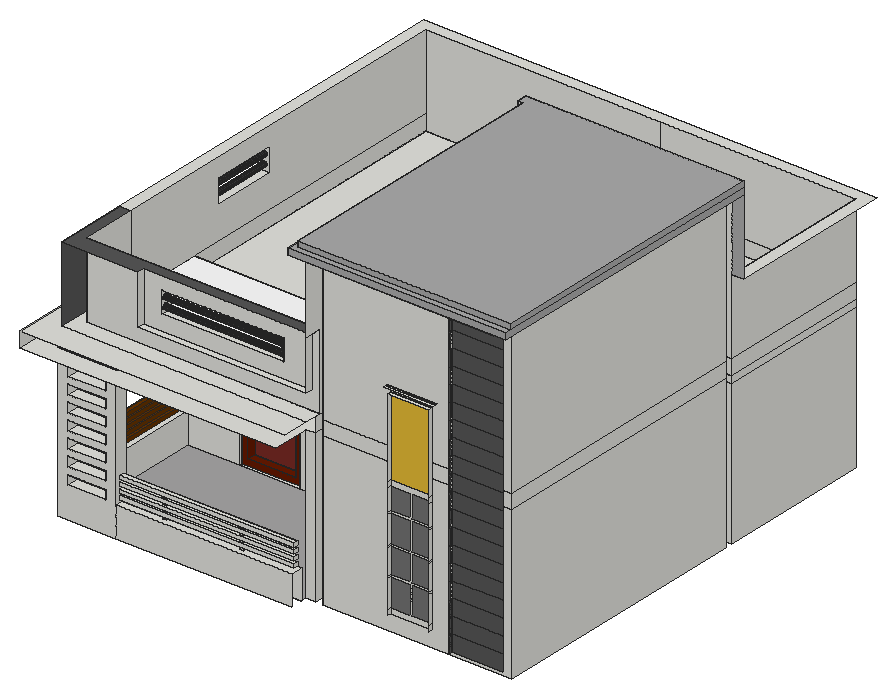
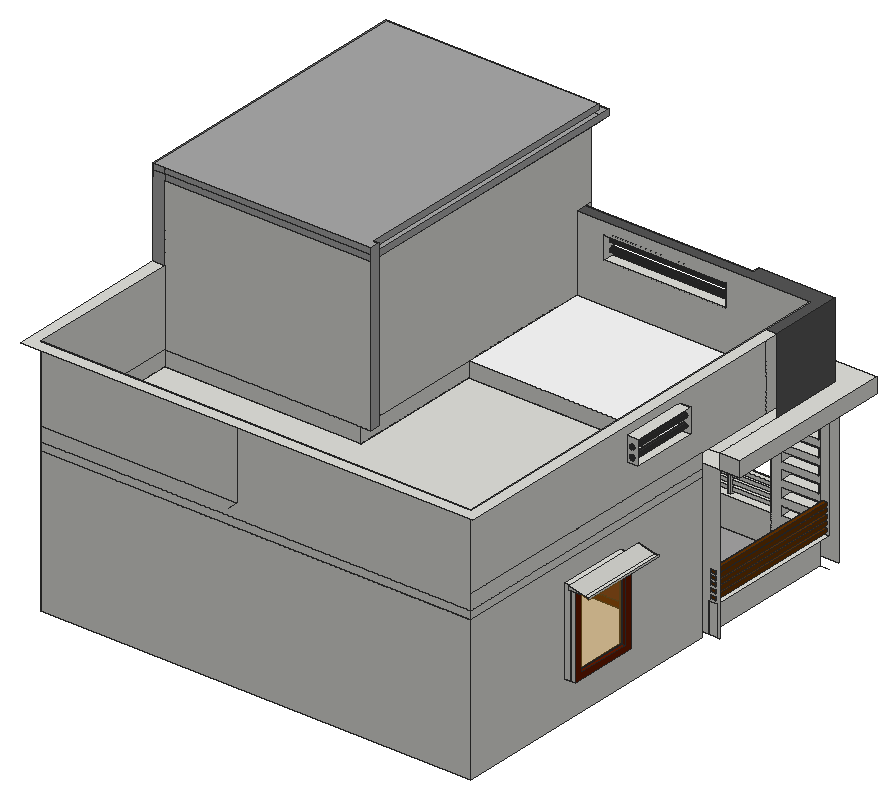
# SketchUp Ruby script. Lengths in inches.
U = 1.inch
M = Sketchup.active_model
def pt(a) = Geom::Point3d.new(a.map { |v| v * U })
def face(e, loops, mat)
  f = e.add_face(loops[0].map { |a| pt(a) })
  loops[1..].each { |l| e.add_face(l.map { |a| pt(a) }).erase! }
  f.material = f.back_material = mat if mat
  f
end
# faces: each face lists its corners as indices into pts; further lists are holes
def faces(e, pts, list, mat = nil) = list.each { |f| face(e, (f[0].is_a?(Array) ? f : [f]).map { |l| l.map { |i| pts[i] } }, mat) }
# xy, xz, yz: faces in a plane at the given z, y or x. An outline is a flat list of corners, or four numbers for a rectangle; further outlines are holes
def ring(l) = l.size == 4 ? [[l[0], l[1]], [l[2], l[1]], [l[2], l[3]], [l[0], l[3]]] : l.each_slice(2).to_a
def flat(e, list, mat, &to3) = list.each { |f| face(e, (f[0].is_a?(Array) ? f : [f]).map { |l| ring(l).map { |u, v| to3.(u, v) } }, mat) }
def xy(e, z, list, mat = nil) = flat(e, list, mat) { |x, y| [x, y, z] }
def xz(e, y, list, mat = nil) = flat(e, list, mat) { |x, z| [x, y, z] }
def yz(e, x, list, mat = nil) = flat(e, list, mat) { |y, z| [x, y, z] }
def lines(e, pts, list) = list.each { |a, b| e.add_line(pt(pts[a]), pt(pts[b])) }
# prism: a flat outline (further loops are holes) pulled along v
def prism(e, loops, v, mat = nil)
  f = face(e, loops, mat); d = Geom::Vector3d.new(v.map { |x| x * U })
  f.pushpull(f.normal.samedirection?(d) ? d.length : -d.length)
end
def box(e, o, s, mat = nil) = prism(e, [[o, [o[0] + s[0], o[1], o[2]], [o[0] + s[0], o[1] + s[1], o[2]], [o[0], o[1] + s[1], o[2]]]], [0, 0, s[2]], mat)
def at(x, y, z, deg = 0) = Geom::Transformation.translation(pt([x, y, z])) * Geom::Transformation.rotation(ORIGIN, Z_AXIS, deg.degrees)
def axes(o, x, y, z) = Geom::Transformation.new([*x, 0, *y, 0, *z, 0, *pt(o).to_a, 1])
def part(name) = M.definitions.add(name)
# library, detail: a bought-in or finely detailed component or shape, given as its bounding box
def library(name, o, s) = part(name).tap { |d| box(d.entities, o, s) }
def detail(e, o, s) = box(e.add_group.entities, o, s)
def put(e, d, t, mat = nil) = e.add_instance(d, t).tap { |i| i.material = mat if mat }
def group(e, t, mat = nil) = e.add_group.tap { |g| g.transformation = t; g.material = mat if mat }.entities
root = M.entities
M.materials.add("[Color B08]").color = [102, 25, 0]
M.materials.add("[Color C08]").color = [102, 51, 0]
M.materials.add("[Color M00]").color = [255, 255, 255]
M.materials.add("[Color M03]").color = [170, 170, 170]
M.materials.add("[Color M05]").color = [114, 114, 114]
M.materials.add("[Color M06]").color = [86, 86, 86]
M.materials.add("[Color M07]").color = [58, 58, 58]
M.materials.add("[Mirror 02]").color = [229, 187, 54]
M.materials.add("[Stone Vein Gray]").color = [166, 165, 165]
M.materials.add("[Translucent Glass Blue]1").color = [223, 149, 22]
M.materials["[Translucent Glass Blue]1"].alpha = 0.5
M.materials.add("[Wood Veneer 01]").color = [120, 43, 37]
c1 = part("Group\#1")
xy(c1.entities,0,[[0,0,48,6.8125]],"[Color B08]")
xy(c1.entities,4.94,[[4.94,0,43.06,6.8125]],"[Color B08]")
xy(c1.entities,79.06,[[4.94,0,43.06,6.8125]],"[Color B08]")
xy(c1.entities,84,[[0,0,48,6.8125]],"[Color B08]")
xz(c1.entities,0,[[[0,0,48,84],[4.94,4.94,43.06,79.06]]],"[Color B08]")
xz(c1.entities,6.8125,[[[0,0,48,84],[4.94,4.94,43.06,79.06]]],"[Color B08]")
xz(c1.entities,6.8125,[[4.94,4.94,43.06,79.06]],"[Wood Veneer 01]")
yz(c1.entities,0,[[0,0,6.8125,84]],"[Color B08]")
yz(c1.entities,4.94,[[0,4.94,6.8125,79.06]],"[Color B08]")
yz(c1.entities,43.06,[[0,4.94,6.8125,79.06]],"[Color B08]")
yz(c1.entities,48,[[0,0,6.8125,84]],"[Color B08]")
c2 = part("Group\#3")
xy(c2.entities,0,[[0,0,48,2.4375]],"[Color B08]")
xy(c2.entities,2.99,[[2.99,0,8.81,2.4375],[8.81,0,14.63,2.4375],[16.47,0,22.65,2.4375],[22.65,0,28.82,2.4375],[30.66,0,45.01,2.4375]],"[Color B08]")
xy(c2.entities,57.01,[[2.99,0,8.81,2.4375],[8.81,0,14.63,2.4375],[16.47,0,22.65,2.4375],[22.65,0,28.82,2.4375],[30.66,0,45.01,2.4375]],"[Color B08]")
xy(c2.entities,60,[[0,0,48,2.4375]],"[Color B08]")
xz(c2.entities,0,[[[0,0,48,60],[30.66,2.99,45.01,57.01],[16.47,2.99,28.82,57.01],[2.99,2.99,14.63,57.01]]],"[Color B08]")
xz(c2.entities,2.4375,[[[0,0,48,60],[30.66,2.99,45.01,57.01],[16.47,2.99,28.82,57.01],[2.99,2.99,14.63,57.01]]],"[Color B08]")
xz(c2.entities,2.4375,[[2.99,2.99,8.81,57.01],[8.81,2.99,14.63,57.01],[16.47,2.99,22.65,57.01],[22.65,2.99,28.82,57.01],[30.66,2.99,45.01,57.01]],"[Translucent Glass Blue]1")
yz(c2.entities,0,[[0,0,2.4375,60]],"[Color B08]")
yz(c2.entities,2.99,[[0,2.99,2.4375,57.01]],"[Color B08]")
yz(c2.entities,14.63,[[0,2.99,2.4375,57.01]],"[Color B08]")
yz(c2.entities,16.47,[[0,2.99,2.4375,57.01]],"[Color B08]")
yz(c2.entities,28.82,[[0,2.99,2.4375,57.01]],"[Color B08]")
yz(c2.entities,30.66,[[0,2.99,2.4375,57.01]],"[Color B08]")
yz(c2.entities,45.01,[[0,2.99,2.4375,57.01]],"[Color B08]")
yz(c2.entities,48,[[0,0,2.4375,60]],"[Color B08]")
c3 = part("Group\#2")
xy(c3.entities,0,[[0,0,23.0625,1.75]],"[Color B08]")
xy(c3.entities,2.13,[[2.13,0,20.93,1.75]],"[Color B08]")
xy(c3.entities,29.8,[[2.13,0,20.93,1.75]],"[Color B08]")
xy(c3.entities,31.9375,[[0,0,23.0625,1.75]],"[Color B08]")
xz(c3.entities,0,[[[0,0,23.0625,31.9375],[2.13,2.13,20.93,29.8]]],"[Color B08]")
xz(c3.entities,1.75,[[[0,0,23.0625,31.9375],[2.13,2.13,20.93,29.8]]],"[Color B08]")
xz(c3.entities,1.75,[[2.13,2.13,20.93,29.8]],"[Translucent Glass Blue]1")
yz(c3.entities,0,[[0,0,1.75,31.9375]],"[Color B08]")
yz(c3.entities,2.13,[[0,2.13,1.75,29.8]],"[Color B08]")
yz(c3.entities,20.93,[[0,2.13,1.75,29.8]],"[Color B08]")
yz(c3.entities,23.0625,[[0,0,1.75,31.9375]],"[Color B08]")
box(root,[62.5625,70.38,249.27],[140.5,3.75,3])
xy(root,213,[[65.72,188.125,113.72,194.125]])
xy(root,213,[[24.85,77.25,203.0625,77.25,203.0625,82.125,210.75,82.125,210.75,188.125,24.85,188.125]],"[Stone Vein Gray]")
xy(root,237,[[[64.19,67.5,203.8125,77.25],[97.86,71.77,100.86,74.2],[158.98,71.77,161.98,74.14]],[97.86,71.77,100.86,74.2],[158.98,71.77,161.98,74.14],[17.6875,77.25,24.85,188.125]])
xy(root,237.55,[[25.89,67.5,55.51,77.25]])
xy(root,239.03,[[19.03,76.6875,22.65,188.125]],"[Color C08]")
xy(root,239.52,[[64.19,70.38,203.0625,74.13]])
xy(root,241.59,[[134.6,188.125,182.6,194.125]])
xy(root,242.03,[[19.03,76.6875,22.65,188.125]],"[Color C08]")
xy(root,242.52,[[64.19,70.38,203.0625,74.13]])
xy(root,243.91,[[19.03,76.375,22.65,188.125]],"[Color C08]")
xy(root,244.22,[[16.0625,276.01,25.0625,331.39]])
xy(root,244.4,[[64.19,70.38,203.0625,74.13]])
xy(root,245.23,[[25.89,67.5,55.51,77.25]])
xy(root,246.91,[[19.03,76.375,22.65,188.125]],"[Color C08]")
xy(root,247.4,[[64.19,70.38,203.0625,74.13]])
xy(root,248.53,[[19.03,77.0625,22.65,188.125]],"[Color C08]")
xy(root,250.86,[[25.89,67.5,55.51,77.25]])
xy(root,251.53,[[19.03,77.0625,22.65,188.125]],"[Color C08]")
xy(root,253.22,[[19.03,77.0625,22.65,188.125]],"[Color C08]")
xy(root,254.15,[[64.19,70.38,64.19,74.13,97.86,74.13,97.86,71.77,100.86,71.77,100.86,74.13,158.98,74.13,158.98,71.77,161.98,71.77,161.98,74.13,203.0625,74.13,203.0625,70.38],[97.86,71.77,100.86,74.13],[158.98,71.77,161.98,74.13],[97.86,74.13,100.86,74.2],[158.98,74.13,161.98,74.14]])
xy(root,256.22,[[19.03,77.0625,22.65,188.125]],"[Color C08]")
xy(root,257.15,[[64.19,70.38,203.0625,74.13]])
xy(root,257.53,[[19.03,76.6875,22.65,188.125]],"[Color C08]")
xy(root,258.55,[[25.89,67.5,55.51,77.25]])
xy(root,260.53,[[19.03,76.6875,22.65,188.125]],"[Color C08]")
xy(root,263.67,[[25.89,67.5,55.51,77.25]])
xy(root,271.36,[[25.89,67.5,55.51,77.25]])
xy(root,276.48,[[25.89,67.5,55.51,77.25]])
xy(root,284.17,[[25.89,67.5,55.51,77.25]])
xy(root,289.3,[[25.89,67.5,55.51,77.25]])
xy(root,296.98,[[25.89,67.5,55.51,77.25]])
xy(root,297,[[65.72,188.125,113.72,194.125]])
xy(root,301.59,[[134.6,188.125,182.6,194.125]])
xy(root,302.11,[[25.89,67.5,55.51,77.25]])
xy(root,309.8,[[25.89,67.5,55.51,77.25]])
xy(root,312.41,[[16.0625,276.01,25.0625,331.39]])
xy(root,313.31,[[0,268.71,16.0625,338.34]])
xy(root,314.92,[[25.89,67.5,55.51,77.25]])
xy(root,322.61,[[25.89,67.5,55.51,77.25]])
xy(root,327,[[25.0625,194.125,25.0625,424.125,367.0625,424.125,367.0625,300.9375,210.75,300.9375,210.75,194.125]])
xy(root,333,[[[0.0625,52.25,0.0625,188.125,210.75,188.125,210.75,82.125,203.0625,82.125,203.0625,52.25],[17.6875,67.5,64.19,77.25]],[17.6875,67.5,25.0625,77.25],[25.0625,67.5,64.19,77.25],[25.0625,194.125,210.75,194.125,210.75,300.9375,367.0625,300.9375,367.0625,424.125,25.0625,424.125]])
xy(root,345,[[0.0625,52.25,210.75,52.25,210.75,73.125,16.0625,73.125,16.0625,188.125,0.0625,188.125],[16.0625,73.125,210.75,73.125,210.75,87.0625,25.0625,87.0625,25.0625,188.125,16.0625,188.125],[203.125,292.82,210.75,300.9375]])
xy(root,345,[[25.0625,87.0625,210.75,194.125]],"[Color M00]")
xy(root,365.8125,[[77.05,73.125,210.75,78.37]])
xy(root,371.23,[[16.0625,216.9,25.0625,269.27]])
xy(root,377.7,[[91.9,78.37,188.65,87.0625]])
xy(root,390.23,[[16.0625,216.9,25.0625,269.27]])
xy(root,391.56,[[279.64,68.125,312.19,71.0625]])
xy(root,395.03,[[276.17,68.125,315.67,70.125],[276.17,70.125,315.67,71.0625]])
xy(root,395.03,[[276.17,71.0625,315.67,72]],"[Color M06]")
xy(root,395.14,[[91.9,78.37,188.65,87.0625]])
xy(root,405,[[16.0625,130.91,25.0625,130.91,25.0625,424.125,367.0625,424.125,367.0625,300.9375,376.0625,300.9375,376.0625,433.125,16.0625,433.125]])
xy(root,405,[[16.0625,73.125,77.05,73.125,77.05,78.37,210.75,78.37,210.75,87.0625,25.0625,87.0625,25.0625,130.91,16.0625,130.91]],"[Color M06]")
xy(root,459,[[216.75,82.125,367.0625,294.9375]])
xy(root,465,[[203.125,64.625,203.125,73.125,264.41,73.125,264.41,70.125,326.55,70.125,326.55,73.125,367.0625,73.125,367.0625,64.625],[264.41,70.125,326.55,71.0625],[264.41,72,326.55,73.125],[216.75,82.125,367.0625,294.9375],[216.75,82.125,367.0625,294.9375]])
xy(root,465,[[203.125,73.125,210.75,292.82]],"[Color M03]")
xy(root,465,[[264.41,71.0625,326.55,72]],"[Color M06]")
xy(root,470,[[203.125,64.625,376.0625,64.625,376.0625,69.375,207.125,69.375,207.125,73.125,203.125,73.125],[203.125,73.125,207.125,292.82]],"[Color M03]")
xy(root,474.75,[[207.125,69.375,376.0625,69.375,376.0625,300.9375,203.125,300.9375,203.125,292.82,207.125,292.82]],"[Color M03]")
xz(root,64.625,[[203.125,465,376.0625,470]],"[Color M03]")
xz(root,67.5,[[[17.6875,213,64.19,333],[25.89,314.92,55.51,322.61],[25.89,302.11,55.51,309.8],[25.89,289.3,55.51,296.98],[25.89,276.48,55.51,284.17],[25.89,263.67,55.51,271.36],[25.89,250.86,55.51,258.55],[25.89,237.55,55.51,245.23]],[64.19,213,203.8125,237]])
xz(root,69.375,[[207.125,470,376.0625,474.75]],"[Color M03]")
xz(root,70.38,[[64.19,239.52,203.0625,242.52],[64.19,244.4,203.0625,247.4],[64.19,254.15,203.0625,257.15]])
xz(root,71.0625,[[279.64,233.67,312.19,233.67,312.19,237.9,296.12,237.9,296.12,260.0625,312.19,260.0625,312.19,261.53,296.12,261.53,296.12,282,312.19,282,312.19,283.47,296.12,283.47,296.12,305.625,312.19,305.625,312.19,307.09,296.12,307.09,296.12,324.48,312.19,324.48,312.19,328.71,279.64,328.71,279.64,324.48,295.68,324.48,295.68,307.09,279.64,307.09,279.64,305.625,295.68,305.625,295.68,283.47,279.64,283.47,279.64,282,295.68,282,295.68,261.53,279.64,261.53,279.64,260.0625,295.68,260.0625,295.68,237.9,279.64,237.9]])
xz(root,71.0625,[[279.64,237.9,295.68,260.0625],[296.12,237.9,312.19,260.0625],[279.64,261.53,295.68,282],[296.12,261.53,312.19,282],[279.64,283.47,295.68,305.625],
  [296.12,283.47,312.19,305.625],[279.64,307.09,295.68,324.48],[296.12,307.09,312.19,324.48]],"[Color M05]")
xz(root,71.0625,[[279.64,328.71,312.19,391.56]],"[Mirror 02]")
xz(root,71.77,[[97.86,237,100.86,254.15],[158.98,237,161.98,254.15]])
xz(root,73.125,[[326.55,221.85,367.0625,234.6],[326.55,234.6,367.0625,247.35],[326.55,247.35,367.0625,260.1],[326.55,260.1,367.0625,272.85],[326.55,272.85,367.0625,285.6],
  [326.55,285.6,367.0625,298.35],[326.55,298.35,367.0625,311.1],[326.55,311.1,367.0625,323.85],[326.55,323.85,367.0625,336.6],[326.55,336.6,367.0625,349.35],
  [326.55,349.35,367.0625,362.1],[326.55,362.1,367.0625,374.85],[326.55,374.85,367.0625,387.6],[326.55,387.6,367.0625,400.35],[326.55,400.35,367.0625,413.1],
  [326.55,413.1,367.0625,425.85],[326.55,425.85,367.0625,438.6],[326.55,438.6,367.0625,451.35],[326.55,451.35,367.0625,465]],"[Color M06]")
xz(root,74.13,[[64.19,239.52,203.0625,242.52],[64.19,244.4,203.0625,247.4],[64.19,254.15,203.0625,257.15]])
xz(root,74.14,[[158.98,237,161.98,254.15]])
xz(root,74.2,[[97.86,237,100.86,254.15]])
xz(root,76.375,[[19.03,243.91,22.65,246.91]],"[Color C08]")
xz(root,76.6875,[[19.03,239.03,22.65,242.03],[19.03,257.53,22.65,260.53]],"[Color C08]")
xz(root,77.0625,[[19.03,248.53,22.65,251.53],[19.03,253.22,22.65,256.22]],"[Color C08]")
xz(root,77.25,[[[24.85,213,64.19,333],[25.89,314.92,55.51,322.61],[25.89,302.11,55.51,309.8],[25.89,289.3,55.51,296.98],[25.89,276.48,55.51,284.17],[25.89,263.67,55.51,271.36],[25.89,250.86,55.51,258.55],[25.89,237.55,55.51,245.23]],[64.19,213,203.8125,237],[17.6875,237,24.85,333]])
xz(root,78.37,[[[77.05,365.8125,210.75,405],[91.9,377.7,188.65,395.14]]])
xz(root,82.125,[[203.0625,213,210.75,333],[216.75,213,367.0625,333],[216.75,333,367.0625,345],[216.75,345,367.0625,459],[216.75,459,367.0625,465]])
xz(root,87.0625,[[[25.0625,345,210.75,405],[91.9,377.7,188.65,395.14]]])
xz(root,188.125,[[[16.0625,213,17.6875,213,17.6875,237,24.85,237,24.85,213,65.72,213,65.72,297,113.72,297,113.72,213,210.75,213,210.75,333,16.0625,333],[134.6,241.59,182.6,301.59],[19.03,257.53,22.65,260.53],[19.03,253.22,22.65,256.22],[19.03,248.53,22.65,251.53],[19.03,243.91,22.65,246.91],[19.03,239.03,22.65,242.03]],[17.6875,213,24.85,237],[0.0625,333,16.0625,345]])
xz(root,188.125,[[19.03,239.03,22.65,242.03],[19.03,243.91,22.65,246.91],[19.03,248.53,22.65,251.53],[19.03,253.22,22.65,256.22],[19.03,257.53,22.65,260.53]],"[Color C08]")
xz(root,194.125,[[[25.0625,213,25.0625,327,210.75,327,210.75,213,113.72,213,113.72,297,65.72,297,65.72,213],[134.6,241.59,182.6,301.59]],[25.0625,327,133.62,333],[133.62,327,144.06,333],[144.06,327,210.75,333],[25.0625,333,210.75,345]])
xz(root,216.27,[[20.63,373.94,21.15,374.01,21.63,374.21,22.05,374.53,22.36,374.94,22.5625,375.42,22.63,375.94,22.5625,376.46,22.36,376.94,22.05,377.35,21.63,377.67,21.15,377.87,20.63,377.94,20.11,377.87,19.63,377.67,19.22,377.35,18.9,376.94,18.7,376.46,18.63,375.94,18.7,375.42,18.9,374.94,19.22,374.53,19.63,374.21,20.11,374.01]],"[Color M07]")
xz(root,216.9,[[[16.0625,371.23,25.0625,390.23],[20.63,381.38,21.15,381.45,21.63,381.65,22.05,381.96,22.36,382.38,22.5625,382.86,22.63,383.38,22.5625,383.9,22.36,384.38,22.05,384.79,21.63,385.11,21.15,385.31,20.63,385.38,20.11,385.31,19.63,385.11,19.22,384.79,18.9,384.38,18.7,383.9,18.63,383.38,18.7,382.86,18.9,382.38,19.22,381.96,19.63,381.65,20.11,381.45]]])
xz(root,268.71,[[0,312.33,0,313.31,16.0625,313.31,16.0625,316.56,3.71,313.31]])
xz(root,269.27,[[[16.0625,371.23,25.0625,390.23],[20.63,373.94,20.11,374.01,19.63,374.21,19.22,374.53,18.9,374.94,18.7,375.42,18.63,375.94,18.7,376.46,18.9,376.94,19.22,377.35,19.63,377.67,20.11,377.87,20.63,377.94,21.15,377.87,21.63,377.67,22.05,377.35,22.36,376.94,22.5625,376.46,22.63,375.94,22.5625,375.42,22.36,374.94,22.05,374.53,21.63,374.21,21.15,374.01],[20.63,381.38,20.11,381.45,19.63,381.65,19.22,381.96,18.9,382.38,18.7,382.86,18.63,383.38,18.7,383.9,18.9,384.38,19.22,384.79,19.63,385.11,20.11,385.31,20.63,385.38,21.15,385.31,21.63,385.11,22.05,384.79,22.36,384.38,22.5625,383.9,22.63,383.38,22.5625,382.86,22.36,382.38,22.05,381.96,21.63,381.65,21.15,381.45]]])
xz(root,269.27,[[20.63,373.94,20.11,374.01,19.63,374.21,19.22,374.53,18.9,374.94,18.7,375.42,18.63,375.94,18.7,376.46,18.9,376.94,19.22,377.35,19.63,377.67,20.11,377.87,20.63,377.94,21.15,377.87,21.63,377.67,22.05,377.35,22.36,376.94,22.5625,376.46,22.63,375.94,22.5625,375.42,22.36,374.94,22.05,374.53,21.63,374.21,21.15,374.01],[20.63,381.38,20.11,381.45,19.63,381.65,19.22,381.96,18.9,382.38,18.7,382.86,18.63,383.38,18.7,383.9,18.9,384.38,19.22,384.79,19.63,385.11,20.11,385.31,20.63,385.38,21.15,385.31,21.63,385.11,22.05,384.79,22.36,384.38,22.5625,383.9,22.63,383.38,22.5625,382.86,22.36,382.38,22.05,381.96,21.63,381.65,21.15,381.45]],"[Color M07]")
xz(root,276.01,[[16.0625,244.22,25.0625,312.41]])
xz(root,292.82,[[203.125,470,207.125,474.75]])
xz(root,292.82,[[203.125,345,210.75,465]],"[Color M03]")
xz(root,294.9375,[[216.75,213,367.0625,333],[216.75,333,367.0625,345],[216.75,345,367.0625,459],[216.75,459,266.67,465],[266.67,459,311.1,465],
  [311.1,459,367.0625,465]])
xz(root,300.9375,[[210.75,213,367.0625,327],[210.75,327,367.0625,333],[210.75,333,367.0625,345],[203.125,345,367.0625,465]])
xz(root,300.9375,[[367.0625,405,376.0625,470],[203.125,465,367.0625,470],[203.125,470,367.0625,474.75],[367.0625,470,376.0625,474.75]],"[Color M03]")
xz(root,331.39,[[16.0625,244.22,25.0625,312.41]])
xz(root,338.34,[[0,312.33,3.71,313.31,16.0625,316.56,16.0625,313.31,0,313.31]])
xz(root,424.125,[[25.0625,213,367.0625,327],[25.0625,327,367.0625,333],[25.0625,333,367.0625,333,367.0625,345,210.75,345,210.75,405,25.0625,405],[210.75,345,367.0625,405]])
yz(root,0,[[268.71,312.33,338.34,313.31]])
yz(root,0.0625,[[52.25,333,188.125,345]])
yz(root,16.0625,[[73.125,345,130.91,405]],"[Color M06]")
yz(root,19.03,[[76.6875,239.03,188.125,242.03],[76.375,243.91,188.125,246.91],[77.0625,248.53,188.125,251.53],[77.0625,253.22,188.125,256.22],[76.6875,257.53,188.125,260.53]],"[Color C08]")
yz(root,22.65,[[76.6875,239.03,188.125,242.03],[76.375,243.91,188.125,246.91],[77.0625,248.53,188.125,251.53],[77.0625,253.22,188.125,256.22],[76.6875,257.53,188.125,260.53]],"[Color C08]")
yz(root,24.85,[[77.25,213,188.125,237]])
yz(root,25.0625,[[[194.125,213,424.125,327],[276.01,244.22,331.39,312.41]],[194.125,327,424.125,333],[194.125,333,424.125,345],[87.0625,345,130.91,405],[[130.91,345,424.125,405],[216.9,371.23,269.27,390.23]]])
yz(root,25.89,[[67.5,237.55,77.25,245.23],[67.5,250.86,77.25,258.55],[67.5,263.67,77.25,271.36],[67.5,276.48,77.25,284.17],[67.5,289.3,77.25,296.98],
  [67.5,302.11,77.25,309.8],[67.5,314.92,77.25,322.61]])
yz(root,55.51,[[67.5,237.55,77.25,245.23],[67.5,250.86,77.25,258.55],[67.5,263.67,77.25,271.36],[67.5,276.48,77.25,284.17],[67.5,289.3,77.25,296.98],
  [67.5,302.11,77.25,309.8],[67.5,314.92,77.25,322.61]])
yz(root,64.19,[[[67.5,237,77.25,333],[70.38,244.4,74.13,247.4],[70.38,239.52,74.13,242.52],[70.38,254.15,74.13,257.15]]])
yz(root,65.72,[[188.125,213,194.125,297]])
yz(root,77.05,[[73.125,365.8125,78.37,405]])
yz(root,91.9,[[[78.37,377.7,87.0625,395.14],[80.3,380.61,79.8,380.67,79.33,380.87,78.93,381.18,78.625,381.58,78.43,382.04,78.37,382.55,78.43,383.05,78.625,383.51,78.93,383.92,79.33,384.22,79.8,384.42,80.3,384.48,80.8,384.42,81.27,384.22,81.67,383.92,81.98,383.51,82.17,383.05,82.24,382.55,82.17,382.04,81.98,381.58,81.67,381.18,81.27,380.87,80.8,380.67],[80.3,387.67,79.8,387.74,79.33,387.93,78.93,388.24,78.625,388.64,78.43,389.11,78.37,389.61,78.43,390.11,78.625,390.58,78.93,390.98,79.33,391.29,79.8,391.48,80.3,391.55,80.8,391.48,81.27,391.29,81.67,390.98,81.98,390.58,82.17,390.11,82.24,389.61,82.17,389.11,81.98,388.64,81.67,388.24,81.27,387.93,80.8,387.74]]])
yz(root,91.9,[[80.3,380.61,79.8,380.67,79.33,380.87,78.93,381.18,78.625,381.58,78.43,382.04,78.37,382.55,78.43,383.05,78.625,383.51,78.93,383.92,79.33,384.22,79.8,384.42,80.3,384.48,80.8,384.42,81.27,384.22,81.67,383.92,81.98,383.51,82.17,383.05,82.24,382.55,82.17,382.04,81.98,381.58,81.67,381.18,81.27,380.87,80.8,380.67],[80.3,387.67,79.8,387.74,79.33,387.93,78.93,388.24,78.625,388.64,78.43,389.11,78.37,389.61,78.43,390.11,78.625,390.58,78.93,390.98,79.33,391.29,79.8,391.48,80.3,391.55,80.8,391.48,81.27,391.29,81.67,390.98,81.98,390.58,82.17,390.11,82.24,389.61,82.17,389.11,81.98,388.64,81.67,388.24,81.27,387.93,80.8,387.74]],"[Color M07]")
yz(root,97.86,[[71.77,237,74.2,254.15]])
yz(root,100.86,[[71.77,237,74.2,254.15]])
yz(root,113.72,[[188.125,213,194.125,297]])
yz(root,134.6,[[188.125,241.59,194.125,301.59]])
yz(root,158.98,[[71.77,237,74.14,254.15]])
yz(root,161.98,[[71.77,237,74.14,254.15]])
yz(root,182.6,[[188.125,241.59,194.125,301.59]])
yz(root,188.65,[[[78.37,377.7,87.0625,395.14],[80.3,387.67,80.8,387.74,81.27,387.93,81.67,388.24,81.98,388.64,82.17,389.11,82.24,389.61,82.17,390.11,81.98,390.58,81.67,390.98,81.27,391.29,80.8,391.48,80.3,391.55,79.8,391.48,79.33,391.29,78.93,390.98,78.625,390.58,78.43,390.11,78.37,389.61,78.43,389.11,78.625,388.64,78.93,388.24,79.33,387.93,79.8,387.74],[80.3,380.61,80.8,380.67,81.27,380.87,81.67,381.18,81.98,381.58,82.17,382.04,82.24,382.55,82.17,383.05,81.98,383.51,81.67,383.92,81.27,384.22,80.8,384.42,80.3,384.48,79.8,384.42,79.33,384.22,78.93,383.92,78.625,383.51,78.43,383.05,78.37,382.55,78.43,382.04,78.625,381.58,78.93,381.18,79.33,380.87,79.8,380.67]]])
yz(root,203.0625,[[70.38,239.52,74.13,242.52],[70.38,244.4,74.13,247.4],[70.38,254.15,74.13,257.15]])
yz(root,203.125,[[292.82,345,300.9375,474.75],[64.625,465,292.82,470]],"[Color M03]")
yz(root,207.125,[[69.375,470,292.82,474.75]],"[Color M03]")
yz(root,210.75,[[82.125,213,188.125,333],[194.125,213,300.9375,327],[194.125,327,300.9375,333],[82.125,333,188.125,345],[194.125,333,300.9375,345],
  [87.0625,345,87.0625,405,73.125,405,73.125,465,292.82,465,292.82,345],[73.125,365.8125,78.37,405]])
yz(root,216.75,[[82.125,213,294.9375,333],[82.125,333,294.9375,345],[82.125,345,294.9375,459],[82.125,459,294.9375,465]])
yz(root,279.64,[[68.125,233.67,71.0625,237.9],[68.125,237.9,71.0625,260.0625],[68.125,260.0625,71.0625,261.53],[68.125,261.53,71.0625,282],[68.125,282,71.0625,283.47],
  [68.125,283.47,71.0625,305.625],[68.125,305.625,71.0625,307.09],[68.125,307.09,71.0625,324.48],[68.125,324.48,71.0625,328.71],[68.125,328.71,71.0625,391.56]])
yz(root,312.19,[[68.125,233.67,71.0625,237.9],[68.125,237.9,71.0625,260.0625],[68.125,260.0625,71.0625,261.53],[68.125,261.53,71.0625,282],[68.125,282,71.0625,283.47],
  [68.125,283.47,71.0625,305.625],[68.125,305.625,71.0625,307.09],[68.125,307.09,71.0625,324.48],[68.125,324.48,71.0625,328.71],[68.125,328.71,71.0625,391.56]])
yz(root,326.55,[[72,221.85,73.125,234.6],[72,234.6,73.125,247.35],[72,247.35,73.125,260.1],[72,260.1,73.125,272.85],[72,272.85,73.125,285.6],
  [72,285.6,73.125,298.35],[72,298.35,73.125,311.1],[72,311.1,73.125,323.85],[72,323.85,73.125,336.6],[72,336.6,73.125,349.35],
  [72,349.35,73.125,362.1],[72,362.1,73.125,374.85],[72,374.85,73.125,387.6],[72,387.6,73.125,400.35],[72,400.35,73.125,413.1],
  [72,413.1,73.125,425.85],[72,425.85,73.125,438.6],[72,438.6,73.125,451.35],[72,451.35,73.125,465]])
yz(root,326.55,[[70.125,221.85,71.0625,234.6],[71.0625,221.85,72,234.6],[70.125,234.6,71.0625,247.35],[71.0625,234.6,72,247.35],[70.125,247.35,71.0625,260.1],
  [71.0625,247.35,72,260.1],[70.125,260.1,71.0625,272.85],[71.0625,260.1,72,272.85],[70.125,272.85,71.0625,285.6],[71.0625,272.85,72,285.6],
  [70.125,285.6,71.0625,298.35],[71.0625,285.6,72,298.35],[70.125,298.35,71.0625,311.1],[71.0625,298.35,72,311.1],[70.125,311.1,71.0625,323.85],
  [71.0625,311.1,72,323.85],[70.125,323.85,71.0625,336.6],[71.0625,323.85,72,336.6],[70.125,336.6,71.0625,349.35],[71.0625,336.6,72,349.35],
  [70.125,349.35,71.0625,362.1],[71.0625,349.35,72,362.1],[70.125,362.1,71.0625,374.85],[71.0625,362.1,72,374.85],[70.125,374.85,71.0625,387.6],
  [71.0625,374.85,72,387.6],[70.125,387.6,71.0625,400.35],[71.0625,387.6,72,400.35],[70.125,400.35,71.0625,413.1],[71.0625,400.35,72,413.1],
  [70.125,413.1,71.0625,425.85],[71.0625,413.1,72,425.85],[70.125,425.85,71.0625,438.6],[71.0625,425.85,72,438.6],[70.125,438.6,71.0625,451.35],
  [71.0625,438.6,72,451.35],[70.125,451.35,71.0625,465],[71.0625,451.35,72,465]],"[Color M06]")
yz(root,367.0625,[[82.125,213,294.9375,333],[300.9375,213,424.125,327],[300.9375,327,424.125,333],[82.125,333,294.9375,345],[300.9375,333,424.125,345],
  [82.125,345,294.9375,459],[300.9375,345,424.125,405],[82.125,459,294.9375,465]])
yz(root,376.0625,[[64.625,465,300.9375,470],[69.375,470,300.9375,474.75]],"[Color M03]")
p = [[3.71,268.71,313.31],[16.0625,268.71,316.56],[16.0625,338.34,316.56],[3.71,338.34,313.31],[0,338.34,312.33],[0,268.71,312.33],
  [20.11,269.27,374.01],[20.63,269.27,373.94],[20.63,216.27,373.94],[20.11,216.27,374.01],[21.15,269.27,374.01],[21.15,216.27,374.01],
  [19.63,269.27,374.21],[19.63,216.27,374.21],[21.63,269.27,374.21],[21.63,216.27,374.21],[19.22,269.27,374.53],[19.22,216.27,374.53],
  [22.05,269.27,374.53],[22.05,216.27,374.53],[18.9,269.27,374.94],[18.9,216.27,374.94],[22.36,269.27,374.94],[22.36,216.27,374.94],
  [18.7,269.27,375.42],[18.7,216.27,375.42],[22.5625,269.27,375.42],[22.5625,216.27,375.42],[18.63,269.27,375.94],[18.63,216.27,375.94],
  [22.63,269.27,375.94],[22.63,216.27,375.94],[18.7,269.27,376.46],[18.7,216.27,376.46],[22.5625,269.27,376.46],[22.5625,216.27,376.46],
  [18.9,269.27,376.94],[18.9,216.27,376.94],[22.36,269.27,376.94],[22.36,216.27,376.94],[19.22,269.27,377.35],[19.22,216.27,377.35],
  [22.05,269.27,377.35],[22.05,216.27,377.35],[19.63,269.27,377.67],[19.63,216.27,377.67],[21.63,269.27,377.67],[21.63,216.27,377.67],
  [20.11,269.27,377.87],[20.11,216.27,377.87],[21.15,269.27,377.87],[21.15,216.27,377.87],[20.63,269.27,377.94],[20.63,216.27,377.94],
  [91.9,79.8,380.67],[91.9,80.3,380.61],[188.65,80.3,380.61],[188.65,79.8,380.67],[91.9,80.8,380.67],[188.65,80.8,380.67],
  [91.9,79.33,380.87],[188.65,79.33,380.87],[91.9,81.27,380.87],[188.65,81.27,380.87],[91.9,78.93,381.18],[188.65,78.93,381.18],
  [91.9,81.67,381.18],[188.65,81.67,381.18],[91.9,78.625,381.58],[188.65,78.625,381.58],[91.9,81.98,381.58],[188.65,81.98,381.58],
  [19.63,269.27,381.65],[20.11,269.27,381.45],[20.11,216.9,381.45],[19.63,216.9,381.65],[20.63,269.27,381.38],[20.63,216.9,381.38],
  [21.15,269.27,381.45],[21.15,216.9,381.45],[21.63,269.27,381.65],[21.63,216.9,381.65],[91.9,78.43,382.04],[188.65,78.43,382.04],
  [91.9,82.17,382.04],[188.65,82.17,382.04],[19.22,269.27,381.96],[19.22,216.9,381.96],[22.05,269.27,381.96],[22.05,216.9,381.96],
  [91.9,78.37,382.55],[188.65,78.37,382.55],[91.9,82.24,382.55],[188.65,82.24,382.55],[18.9,269.27,382.38],[18.9,216.9,382.38],
  [22.36,269.27,382.38],[22.36,216.9,382.38],[18.7,269.27,382.86],[18.7,216.9,382.86],[22.5625,269.27,382.86],[22.5625,216.9,382.86],
  [91.9,78.43,383.05],[188.65,78.43,383.05],[91.9,82.17,383.05],[188.65,82.17,383.05],[18.63,269.27,383.38],[18.63,216.9,383.38],
  [22.63,269.27,383.38],[22.63,216.9,383.38],[91.9,78.625,383.51],[188.65,78.625,383.51],[91.9,81.98,383.51],[188.65,81.98,383.51],
  [18.7,269.27,383.9],[18.7,216.9,383.9],[22.5625,269.27,383.9],[22.5625,216.9,383.9],[91.9,78.93,383.92],[188.65,78.93,383.92],
  [91.9,81.67,383.92],[188.65,81.67,383.92],[91.9,79.33,384.22],[188.65,79.33,384.22],[91.9,81.27,384.22],[188.65,81.27,384.22],
  [18.9,269.27,384.38],[18.9,216.9,384.38],[22.36,269.27,384.38],[22.36,216.9,384.38],[91.9,79.8,384.42],[188.65,79.8,384.42],
  [91.9,80.8,384.42],[188.65,80.8,384.42],[91.9,80.3,384.48],[188.65,80.3,384.48],[19.22,269.27,384.79],[19.22,216.9,384.79],
  [22.05,269.27,384.79],[22.05,216.9,384.79],[19.63,269.27,385.11],[19.63,216.9,385.11],[21.63,269.27,385.11],[21.63,216.9,385.11],
  [20.11,269.27,385.31],[20.11,216.9,385.31],[21.15,269.27,385.31],[21.15,216.9,385.31],[20.63,269.27,385.38],[20.63,216.9,385.38],
  [91.9,79.33,387.93],[91.9,79.8,387.74],[188.65,79.8,387.74],[188.65,79.33,387.93],[91.9,80.3,387.67],[188.65,80.3,387.67],
  [91.9,80.8,387.74],[188.65,80.8,387.74],[91.9,81.27,387.93],[188.65,81.27,387.93],[91.9,78.93,388.24],[188.65,78.93,388.24],
  [91.9,81.67,388.24],[188.65,81.67,388.24],[91.9,78.625,388.64],[188.65,78.625,388.64],[91.9,81.98,388.64],[188.65,81.98,388.64],
  [91.9,78.43,389.11],[188.65,78.43,389.11],[91.9,82.17,389.11],[188.65,82.17,389.11],[91.9,78.37,389.61],[188.65,78.37,389.61],
  [91.9,82.24,389.61],[188.65,82.24,389.61],[91.9,78.43,390.11],[188.65,78.43,390.11],[91.9,82.17,390.11],[188.65,82.17,390.11],
  [91.9,78.625,390.58],[188.65,78.625,390.58],[91.9,81.98,390.58],[188.65,81.98,390.58],[91.9,78.93,390.98],[188.65,78.93,390.98],
  [91.9,81.67,390.98],[188.65,81.67,390.98],[91.9,79.33,391.29],[188.65,79.33,391.29],[91.9,81.27,391.29],[188.65,81.27,391.29],
  [91.9,79.8,391.48],[188.65,79.8,391.48],[91.9,80.8,391.48],[188.65,80.8,391.48],[91.9,80.3,391.55],[188.65,80.3,391.55],
  [24.85,77.25,213],[17.6875,77.25,213],[210.75,424.125,345],[210.75,433.125,345]]
faces(root,p,[[0,1,2,3,4,5]])
faces(root,p,[[6,7,8,9],[7,10,11,8],[12,6,9,13],[10,14,15,11],[16,12,13,17],[14,18,19,15],[20,16,17,21],[18,22,23,19],
  [24,20,21,25],[22,26,27,23],[28,24,25,29],[26,30,31,27],[32,28,29,33],[30,34,35,31],[36,32,33,37],[34,38,39,35],
  [40,36,37,41],[38,42,43,39],[44,40,41,45],[42,46,47,43],[48,44,45,49],[46,50,51,47],[52,48,49,53],[50,52,53,51],
  [54,55,56,57],[55,58,59,56],[60,54,57,61],[58,62,63,59],[64,60,61,65],[62,66,67,63],[68,64,65,69],[66,70,71,67],
  [72,73,74,75],[73,76,77,74],[76,78,79,77],[78,80,81,79],[82,68,69,83],[70,84,85,71],[86,72,75,87],[80,88,89,81],
  [90,82,83,91],[84,92,93,85],[94,86,87,95],[88,96,97,89],[98,94,95,99],[96,100,101,97],[102,90,91,103],[92,104,105,93],
  [106,98,99,107],[100,108,109,101],[110,102,103,111],[104,112,113,105],[114,106,107,115],[108,116,117,109],[118,110,111,119],[112,120,121,113],
  [122,118,119,123],[120,124,125,121],[126,114,115,127],[116,128,129,117],[130,122,123,131],[124,132,133,125],[134,130,131,135],[132,134,135,133],
  [136,126,127,137],[128,138,139,129],[140,136,137,141],[138,142,143,139],[144,140,141,145],[142,146,147,143],[148,144,145,149],[146,148,149,147],
  [150,151,152,153],[151,154,155,152],[154,156,157,155],[156,158,159,157],[160,150,153,161],[158,162,163,159],[164,160,161,165],[162,166,167,163],
  [168,164,165,169],[166,170,171,167],[172,168,169,173],[170,174,175,171],[176,172,173,177],[174,178,179,175],[180,176,177,181],[178,182,183,179],
  [184,180,181,185],[182,186,187,183],[188,184,185,189],[186,190,191,187],[192,188,189,193],[190,194,195,191],[196,192,193,197],[194,196,197,195]],"[Color M07]")
lines(root,p,[[198,199],[200,201]])
put(root,c1,at(65.72,190.5,213))
put(root,c2,at(134.6,188.125,241.59))
put(root,c3,axes([16.0625,331.39,244.22],[0,-2.40108,0],[2,0,0],[0,0,2.13503]))
